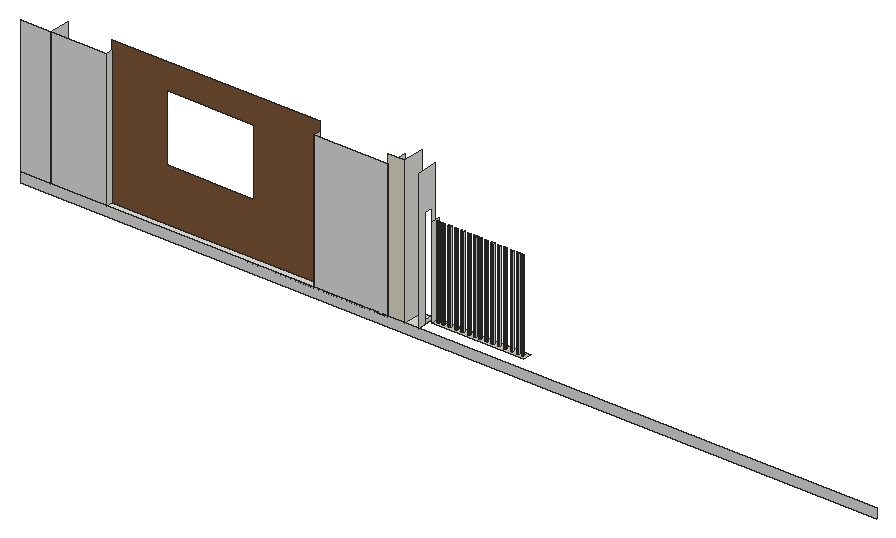
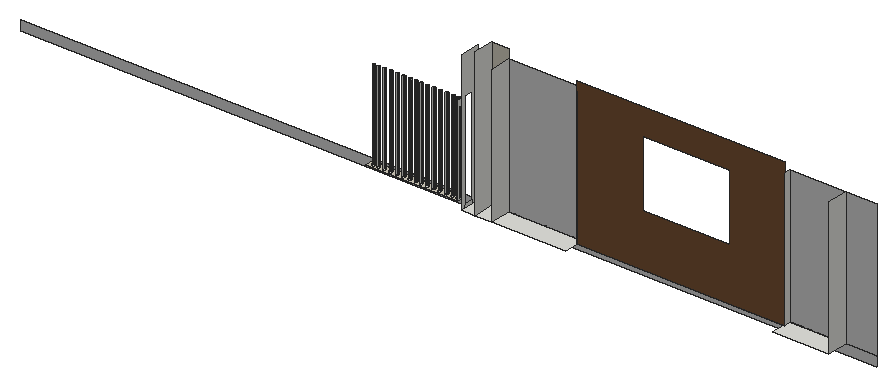
# SketchUp Ruby script. Lengths in inches.
U = 1.inch
M = Sketchup.active_model
def pt(a) = Geom::Point3d.new(a.map { |v| v * U })
def face(e, loops, mat)
  f = e.add_face(loops[0].map { |a| pt(a) })
  loops[1..].each { |l| e.add_face(l.map { |a| pt(a) }).erase! }
  f.material = f.back_material = mat if mat
  f
end
# faces: each face lists its corners as indices into pts; further lists are holes
def faces(e, pts, list, mat = nil) = list.each { |f| face(e, (f[0].is_a?(Array) ? f : [f]).map { |l| l.map { |i| pts[i] } }, mat) }
# xy, xz, yz: faces in a plane at the given z, y or x. An outline is a flat list of corners, or four numbers for a rectangle; further outlines are holes
def ring(l) = l.size == 4 ? [[l[0], l[1]], [l[2], l[1]], [l[2], l[3]], [l[0], l[3]]] : l.each_slice(2).to_a
def flat(e, list, mat, &to3) = list.each { |f| face(e, (f[0].is_a?(Array) ? f : [f]).map { |l| ring(l).map { |u, v| to3.(u, v) } }, mat) }
def xy(e, z, list, mat = nil) = flat(e, list, mat) { |x, y| [x, y, z] }
def xz(e, y, list, mat = nil) = flat(e, list, mat) { |x, z| [x, y, z] }
def yz(e, x, list, mat = nil) = flat(e, list, mat) { |y, z| [x, y, z] }
def lines(e, pts, list) = list.each { |a, b| e.add_line(pt(pts[a]), pt(pts[b])) }
# prism: a flat outline (further loops are holes) pulled along v
def prism(e, loops, v, mat = nil)
  f = face(e, loops, mat); d = Geom::Vector3d.new(v.map { |x| x * U })
  f.pushpull(f.normal.samedirection?(d) ? d.length : -d.length)
end
def box(e, o, s, mat = nil) = prism(e, [[o, [o[0] + s[0], o[1], o[2]], [o[0] + s[0], o[1] + s[1], o[2]], [o[0], o[1] + s[1], o[2]]]], [0, 0, s[2]], mat)
def at(x, y, z, deg = 0) = Geom::Transformation.translation(pt([x, y, z])) * Geom::Transformation.rotation(ORIGIN, Z_AXIS, deg.degrees)
def axes(o, x, y, z) = Geom::Transformation.new([*x, 0, *y, 0, *z, 0, *pt(o).to_a, 1])
def part(name) = M.definitions.add(name)
# library, detail: a bought-in or finely detailed component or shape, given as its bounding box
def library(name, o, s) = part(name).tap { |d| box(d.entities, o, s) }
def detail(e, o, s) = box(e.add_group.entities, o, s)
def put(e, d, t, mat = nil) = e.add_instance(d, t).tap { |i| i.material = mat if mat }
def group(e, t, mat = nil) = e.add_group.tap { |g| g.transformation = t; g.material = mat if mat }.entities
root = M.entities
M.materials.add("[Cladding Siding White]").color = [207, 207, 207]
M.materials.add("[Formica Graystone]").color = [209, 204, 189]
M.materials.add("[Sandstone]").color = [118, 81, 52]
xy(root,9,[[28.1,1.67,80.35,21.38],[80.35,1.67,273.1875,8.25],[273.1875,1.67,342.51,21.38],[342.51,1.67,357.9375,21.38],[357.9375,1.67,370.65,21.38]])
xy(root,12.5,[[380.14,12.51,379.82,12.55,379.52,12.67,379.26,12.875,379.06,13.13,378.94,13.43,378.89,13.76,378.94,14.08,379.06,14.38,379.26,14.64,379.52,14.84,379.82,14.96,380.14,15.01,380.47,14.96,380.77,14.84,381.03,14.64,381.23,14.38,381.35,14.08,381.39,13.76,381.35,13.43,381.23,13.13,381.03,12.875,380.77,12.67,380.47,12.55],[384.7,12.51,384.38,12.55,384.08,12.67,383.82,12.875,383.62,13.13,383.49,13.43,383.45,13.76,383.49,14.08,383.62,14.38,383.82,14.64,384.08,14.84,384.38,14.96,384.7,15.01,385.03,14.96,385.33,14.84,385.59,14.64,385.78,14.38,385.91,14.08,385.95,13.76,385.91,13.43,385.78,13.13,385.59,12.875,385.33,12.67,385.03,12.55],[390.45,12.51,390.13,12.55,389.83,12.67,389.57,12.875,389.37,13.13,389.24,13.43,389.2,13.76,389.24,14.08,389.37,14.38,389.57,14.64,389.83,14.84,390.13,14.96,390.45,15.01,390.78,14.96,391.08,14.84,391.34,14.64,391.53,14.38,391.66,14.08,391.7,13.76,391.66,13.43,391.53,13.13,391.34,12.875,391.08,12.67,390.78,12.55],[396.95,12.51,396.63,12.55,396.33,12.67,396.07,12.875,395.87,13.13,395.74,13.43,395.7,13.76,395.74,14.08,395.87,14.38,396.07,14.64,396.33,14.84,396.63,14.96,396.95,15.01,397.28,14.96,397.58,14.84,397.84,14.64,398.03,14.38,398.16,14.08,398.2,13.76,398.16,13.43,398.03,13.13,397.84,12.875,397.58,12.67,397.28,12.55],[402.58,12.51,402.25,12.55,401.95,12.67,401.69,12.875,401.49,13.13,401.37,13.43,401.33,13.76,401.37,14.08,401.49,14.38,401.69,14.64,401.95,14.84,402.25,14.96,402.58,15.01,402.9,14.96,403.2,14.84,403.46,14.64,403.66,14.38,403.78,14.08,403.83,13.76,403.78,13.43,403.66,13.13,403.46,12.875,403.2,12.67,402.9,12.55],
  [408.45,12.51,408.13,12.55,407.83,12.67,407.57,12.875,407.37,13.13,407.24,13.43,407.2,13.76,407.24,14.08,407.37,14.38,407.57,14.64,407.83,14.84,408.13,14.96,408.45,15.01,408.78,14.96,409.08,14.84,409.34,14.64,409.53,14.38,409.66,14.08,409.7,13.76,409.66,13.43,409.53,13.13,409.34,12.875,409.08,12.67,408.78,12.55],[414.01,12.51,413.69,12.55,413.39,12.67,413.13,12.875,412.93,13.13,412.81,13.43,412.76,13.76,412.81,14.08,412.93,14.38,413.13,14.64,413.39,14.84,413.69,14.96,414.01,15.01,414.34,14.96,414.64,14.84,414.9,14.64,415.1,14.38,415.22,14.08,415.26,13.76,415.22,13.43,415.1,13.13,414.9,12.875,414.64,12.67,414.34,12.55],[418.89,12.51,418.57,12.55,418.26,12.67,418.01,12.875,417.81,13.13,417.68,13.43,417.64,13.76,417.68,14.08,417.81,14.38,418.01,14.64,418.26,14.84,418.57,14.96,418.89,15.01,419.21,14.96,419.51,14.84,419.77,14.64,419.97,14.38,420.1,14.08,420.14,13.76,420.1,13.43,419.97,13.13,419.77,12.875,419.51,12.67,419.21,12.55],[424.64,12.51,424.32,12.55,424.01,12.67,423.76,12.875,423.56,13.13,423.43,13.43,423.39,13.76,423.43,14.08,423.56,14.38,423.76,14.64,424.01,14.84,424.32,14.96,424.64,15.01,424.96,14.96,425.26,14.84,425.52,14.64,425.72,14.38,425.85,14.08,425.89,13.76,425.85,13.43,425.72,13.13,425.52,12.875,425.26,12.67,424.96,12.55],[430.51,12.51,430.19,12.55,429.89,12.67,429.63,12.875,429.43,13.13,429.31,13.43,429.26,13.76,429.31,14.08,429.43,14.38,429.63,14.64,429.89,14.84,430.19,14.96,430.51,15.01,430.84,14.96,431.14,14.84,431.4,14.64,431.6,14.38,431.72,14.08,431.76,13.76,431.72,13.43,431.6,13.13,431.4,12.875,431.14,12.67,430.84,12.55],
  [436.2,12.51,435.88,12.55,435.58,12.67,435.32,12.875,435.12,13.13,434.99,13.43,434.95,13.76,434.99,14.08,435.12,14.38,435.32,14.64,435.58,14.84,435.88,14.96,436.2,15.01,436.53,14.96,436.83,14.84,437.09,14.64,437.28,14.38,437.41,14.08,437.45,13.76,437.41,13.43,437.28,13.13,437.09,12.875,436.83,12.67,436.53,12.55],[442.45,12.51,442.13,12.55,441.83,12.67,441.57,12.875,441.37,13.13,441.24,13.43,441.2,13.76,441.24,14.08,441.37,14.38,441.57,14.64,441.83,14.84,442.13,14.96,442.45,15.01,442.78,14.96,443.08,14.84,443.34,14.64,443.53,14.38,443.66,14.08,443.7,13.76,443.66,13.43,443.53,13.13,443.34,12.875,443.08,12.67,442.78,12.55],[448.45,12.51,448.13,12.55,447.83,12.67,447.57,12.875,447.37,13.13,447.24,13.43,447.2,13.76,447.24,14.08,447.37,14.38,447.57,14.64,447.83,14.84,448.13,14.96,448.45,15.01,448.78,14.96,449.08,14.84,449.34,14.64,449.53,14.38,449.66,14.08,449.7,13.76,449.66,13.43,449.53,13.13,449.34,12.875,449.08,12.67,448.78,12.55],[453.95,12.51,453.63,12.55,453.33,12.67,453.07,12.875,452.87,13.13,452.74,13.43,452.7,13.76,452.74,14.08,452.87,14.38,453.07,14.64,453.33,14.84,453.63,14.96,453.95,15.01,454.28,14.96,454.58,14.84,454.84,14.64,455.03,14.38,455.16,14.08,455.2,13.76,455.16,13.43,455.03,13.13,454.84,12.875,454.58,12.67,454.28,12.55],[458.64,12.51,458.32,12.55,458.01,12.67,457.76,12.875,457.56,13.13,457.43,13.43,457.39,13.76,457.43,14.08,457.56,14.38,457.76,14.64,458.01,14.84,458.32,14.96,458.64,15.01,458.96,14.96,459.26,14.84,459.52,14.64,459.72,14.38,459.85,14.08,459.89,13.76,459.85,13.43,459.72,13.13,459.52,12.875,459.26,12.67,458.96,12.55]])
xy(root,12.5,[[[377.34,9.54,462.5,17.41],[380.14,12.51,379.82,12.55,379.52,12.67,379.26,12.875,379.06,13.13,378.94,13.43,378.89,13.76,378.94,14.08,379.06,14.38,379.26,14.64,379.52,14.84,379.82,14.96,380.14,15.01,380.47,14.96,380.77,14.84,381.03,14.64,381.23,14.38,381.35,14.08,381.39,13.76,381.35,13.43,381.23,13.13,381.03,12.875,380.77,12.67,380.47,12.55],[458.64,12.51,458.32,12.55,458.01,12.67,457.76,12.875,457.56,13.13,457.43,13.43,457.39,13.76,457.43,14.08,457.56,14.38,457.76,14.64,458.01,14.84,458.32,14.96,458.64,15.01,458.96,14.96,459.26,14.84,459.52,14.64,459.72,14.38,459.85,14.08,459.89,13.76,459.85,13.43,459.72,13.13,459.52,12.875,459.26,12.67,458.96,12.55],[384.7,12.51,384.38,12.55,384.08,12.67,383.82,12.875,383.62,13.13,383.49,13.43,383.45,13.76,383.49,14.08,383.62,14.38,383.82,14.64,384.08,14.84,384.38,14.96,384.7,15.01,385.03,14.96,385.33,14.84,385.59,14.64,385.78,14.38,385.91,14.08,385.95,13.76,385.91,13.43,385.78,13.13,385.59,12.875,385.33,12.67,385.03,12.55],[453.95,12.51,453.63,12.55,453.33,12.67,453.07,12.875,452.87,13.13,452.74,13.43,452.7,13.76,452.74,14.08,452.87,14.38,453.07,14.64,453.33,14.84,453.63,14.96,453.95,15.01,454.28,14.96,454.58,14.84,454.84,14.64,455.03,14.38,455.16,14.08,455.2,13.76,455.16,13.43,455.03,13.13,454.84,12.875,454.58,12.67,454.28,12.55],[390.45,12.51,390.13,12.55,389.83,12.67,389.57,12.875,389.37,13.13,389.24,13.43,389.2,13.76,389.24,14.08,389.37,14.38,389.57,14.64,389.83,14.84,390.13,14.96,390.45,15.01,390.78,14.96,391.08,14.84,391.34,14.64,391.53,14.38,391.66,14.08,391.7,13.76,391.66,13.43,391.53,13.13,391.34,12.875,391.08,12.67,390.78,12.55],[448.45,12.51,448.13,12.55,447.83,12.67,447.57,12.875,447.37,13.13,447.24,13.43,447.2,13.76,447.24,14.08,447.37,14.38,447.57,14.64,447.83,14.84,448.13,14.96,448.45,15.01,448.78,14.96,449.08,14.84,449.34,14.64,449.53,14.38,449.66,14.08,449.7,13.76,449.66,13.43,449.53,13.13,449.34,12.875,449.08,12.67,448.78,12.55],[396.95,12.51,396.63,12.55,396.33,12.67,396.07,12.875,395.87,13.13,395.74,13.43,395.7,13.76,395.74,14.08,395.87,14.38,396.07,14.64,396.33,14.84,396.63,14.96,396.95,15.01,397.28,14.96,397.58,14.84,397.84,14.64,398.03,14.38,398.16,14.08,398.2,13.76,398.16,13.43,398.03,13.13,397.84,12.875,397.58,12.67,397.28,12.55],[442.45,12.51,442.13,12.55,441.83,12.67,441.57,12.875,441.37,13.13,441.24,13.43,441.2,13.76,441.24,14.08,441.37,14.38,441.57,14.64,441.83,14.84,442.13,14.96,442.45,15.01,442.78,14.96,443.08,14.84,443.34,14.64,443.53,14.38,443.66,14.08,443.7,13.76,443.66,13.43,443.53,13.13,443.34,12.875,443.08,12.67,442.78,12.55],[402.58,12.51,402.25,12.55,401.95,12.67,401.69,12.875,401.49,13.13,401.37,13.43,401.33,13.76,401.37,14.08,401.49,14.38,401.69,14.64,401.95,14.84,402.25,14.96,402.58,15.01,402.9,14.96,403.2,14.84,403.46,14.64,403.66,14.38,403.78,14.08,403.83,13.76,403.78,13.43,403.66,13.13,403.46,12.875,403.2,12.67,402.9,12.55],[436.2,12.51,435.88,12.55,435.58,12.67,435.32,12.875,435.12,13.13,434.99,13.43,434.95,13.76,434.99,14.08,435.12,14.38,435.32,14.64,435.58,14.84,435.88,14.96,436.2,15.01,436.53,14.96,436.83,14.84,437.09,14.64,437.28,14.38,437.41,14.08,437.45,13.76,437.41,13.43,437.28,13.13,437.09,12.875,436.83,12.67,436.53,12.55],[408.45,12.51,408.13,12.55,407.83,12.67,407.57,12.875,407.37,13.13,407.24,13.43,407.2,13.76,407.24,14.08,407.37,14.38,407.57,14.64,407.83,14.84,408.13,14.96,408.45,15.01,408.78,14.96,409.08,14.84,409.34,14.64,409.53,14.38,409.66,14.08,409.7,13.76,409.66,13.43,409.53,13.13,409.34,12.875,409.08,12.67,408.78,12.55],[430.51,12.51,430.19,12.55,429.89,12.67,429.63,12.875,429.43,13.13,429.31,13.43,429.26,13.76,429.31,14.08,429.43,14.38,429.63,14.64,429.89,14.84,430.19,14.96,430.51,15.01,430.84,14.96,431.14,14.84,431.4,14.64,431.6,14.38,431.72,14.08,431.76,13.76,431.72,13.43,431.6,13.13,431.4,12.875,431.14,12.67,430.84,12.55],[414.01,12.51,413.69,12.55,413.39,12.67,413.13,12.875,412.93,13.13,412.81,13.43,412.76,13.76,412.81,14.08,412.93,14.38,413.13,14.64,413.39,14.84,413.69,14.96,414.01,15.01,414.34,14.96,414.64,14.84,414.9,14.64,415.1,14.38,415.22,14.08,415.26,13.76,415.22,13.43,415.1,13.13,414.9,12.875,414.64,12.67,414.34,12.55],[418.89,12.51,418.57,12.55,418.26,12.67,418.01,12.875,417.81,13.13,417.68,13.43,417.64,13.76,417.68,14.08,417.81,14.38,418.01,14.64,418.26,14.84,418.57,14.96,418.89,15.01,419.21,14.96,419.51,14.84,419.77,14.64,419.97,14.38,420.1,14.08,420.14,13.76,420.1,13.43,419.97,13.13,419.77,12.875,419.51,12.67,419.21,12.55],[424.64,12.51,424.32,12.55,424.01,12.67,423.76,12.875,423.56,13.13,423.43,13.43,423.39,13.76,423.43,14.08,423.56,14.38,423.76,14.64,424.01,14.84,424.32,14.96,424.64,15.01,424.96,14.96,425.26,14.84,425.52,14.64,425.72,14.38,425.85,14.08,425.89,13.76,425.85,13.43,425.72,13.13,425.52,12.875,425.26,12.67,424.96,12.55]]],"[Formica Graystone]")
xz(root,1.67,[[0,0,797.12,9],[0,9,28.1,136.125],[28.1,9,80.35,136.125],[273.1875,9,342.51,136.125]],"[Cladding Siding White]")
xz(root,1.67,[[342.51,9,357.9375,145.125]],"[Formica Graystone]")
xz(root,8.25,[[[80.35,9,273.1875,145.125],[130.9,58.17,212.59,120.61]]],"[Sandstone]")
yz(root,28.1,[[1.67,9,21.38,136.125]])
yz(root,80.35,[[1.67,9,8.25,136.125]])
yz(root,273.1875,[[1.67,9,8.25,136.125]])
yz(root,342.51,[[1.67,9,21.38,136.125]])
yz(root,357.9375,[[1.67,9,21.38,145.125]])
yz(root,370.65,[[1.67,9,9.54,9,9.54,102.25,17.41,102.25,17.41,9,21.38,9,21.38,138.11,1.67,138.11],[9.54,9,17.41,12.5]])
yz(root,377.34,[[9.54,12.5,17.41,96.37]])
p = [[379.52,12.67,12.5],[379.82,12.55,12.5],[379.82,12.55,96.37],[379.52,12.67,96.37],[380.14,12.51,12.5],[380.14,12.51,96.37],
  [380.47,12.55,12.5],[380.47,12.55,96.37],[380.77,12.67,12.5],[380.77,12.67,96.37],[384.08,12.67,12.5],[384.38,12.55,12.5],
  [384.38,12.55,96.37],[384.08,12.67,96.37],[384.7,12.51,12.5],[384.7,12.51,96.37],[385.03,12.55,12.5],[385.03,12.55,96.37],
  [385.33,12.67,12.5],[385.33,12.67,96.37],[389.83,12.67,12.5],[390.13,12.55,12.5],[390.13,12.55,96.37],[389.83,12.67,96.37],
  [390.45,12.51,12.5],[390.45,12.51,96.37],[390.78,12.55,12.5],[390.78,12.55,96.37],[391.08,12.67,12.5],[391.08,12.67,96.37],
  [396.33,12.67,12.5],[396.63,12.55,12.5],[396.63,12.55,96.37],[396.33,12.67,96.37],[396.95,12.51,12.5],[396.95,12.51,96.37],
  [397.28,12.55,12.5],[397.28,12.55,96.37],[397.58,12.67,12.5],[397.58,12.67,96.37],[401.95,12.67,12.5],[402.25,12.55,12.5],
  [402.25,12.55,96.37],[401.95,12.67,96.37],[402.58,12.51,12.5],[402.58,12.51,96.37],[402.9,12.55,12.5],[402.9,12.55,96.37],
  [403.2,12.67,12.5],[403.2,12.67,96.37],[407.83,12.67,12.5],[408.13,12.55,12.5],[408.13,12.55,96.37],[407.83,12.67,96.37],
  [408.45,12.51,12.5],[408.45,12.51,96.37],[408.78,12.55,12.5],[408.78,12.55,96.37],[409.08,12.67,12.5],[409.08,12.67,96.37],
  [413.39,12.67,12.5],[413.69,12.55,12.5],[413.69,12.55,96.37],[413.39,12.67,96.37],[414.01,12.51,12.5],[414.01,12.51,96.37],
  [414.34,12.55,12.5],[414.34,12.55,96.37],[414.64,12.67,12.5],[414.64,12.67,96.37],[418.26,12.67,12.5],[418.57,12.55,12.5],
  [418.57,12.55,96.37],[418.26,12.67,96.37],[418.89,12.51,12.5],[418.89,12.51,96.37],[419.21,12.55,12.5],[419.21,12.55,96.37],
  [419.51,12.67,12.5],[419.51,12.67,96.37],[424.01,12.67,12.5],[424.32,12.55,12.5],[424.32,12.55,96.37],[424.01,12.67,96.37],
  [424.64,12.51,12.5],[424.64,12.51,96.37],[424.96,12.55,12.5],[424.96,12.55,96.37],[425.26,12.67,12.5],[425.26,12.67,96.37],
  [429.89,12.67,12.5],[430.19,12.55,12.5],[430.19,12.55,96.37],[429.89,12.67,96.37],[430.51,12.51,12.5],[430.51,12.51,96.37],
  [430.84,12.55,12.5],[430.84,12.55,96.37],[431.14,12.67,12.5],[431.14,12.67,96.37],[435.58,12.67,12.5],[435.88,12.55,12.5],
  [435.88,12.55,96.37],[435.58,12.67,96.37],[436.2,12.51,12.5],[436.2,12.51,96.37],[436.53,12.55,12.5],[436.53,12.55,96.37],
  [436.83,12.67,12.5],[436.83,12.67,96.37],[441.83,12.67,12.5],[442.13,12.55,12.5],[442.13,12.55,96.37],[441.83,12.67,96.37],
  [442.45,12.51,12.5],[442.45,12.51,96.37],[442.78,12.55,12.5],[442.78,12.55,96.37],[443.08,12.67,12.5],[443.08,12.67,96.37],
  [447.83,12.67,12.5],[448.13,12.55,12.5],[448.13,12.55,96.37],[447.83,12.67,96.37],[448.45,12.51,12.5],[448.45,12.51,96.37],
  [448.78,12.55,12.5],[448.78,12.55,96.37],[449.08,12.67,12.5],[449.08,12.67,96.37],[453.33,12.67,12.5],[453.63,12.55,12.5],
  [453.63,12.55,96.37],[453.33,12.67,96.37],[453.95,12.51,12.5],[453.95,12.51,96.37],[454.28,12.55,12.5],[454.28,12.55,96.37],
  [454.58,12.67,12.5],[454.58,12.67,96.37],[458.01,12.67,12.5],[458.32,12.55,12.5],[458.32,12.55,96.37],[458.01,12.67,96.37],
  [458.64,12.51,12.5],[458.64,12.51,96.37],[458.96,12.55,12.5],[458.96,12.55,96.37],[459.26,12.67,12.5],[459.26,12.67,96.37],
  [379.26,12.875,12.5],[379.26,12.875,96.37],[381.03,12.875,12.5],[381.03,12.875,96.37],[383.82,12.875,12.5],[383.82,12.875,96.37],
  [385.59,12.875,12.5],[385.59,12.875,96.37],[389.57,12.875,12.5],[389.57,12.875,96.37],[391.34,12.875,12.5],[391.34,12.875,96.37],
  [396.07,12.875,12.5],[396.07,12.875,96.37],[397.84,12.875,12.5],[397.84,12.875,96.37],[401.69,12.875,12.5],[401.69,12.875,96.37],
  [403.46,12.875,12.5],[403.46,12.875,96.37],[407.57,12.875,12.5],[407.57,12.875,96.37],[409.34,12.875,12.5],[409.34,12.875,96.37],
  [413.13,12.875,12.5],[413.13,12.875,96.37],[414.9,12.875,12.5],[414.9,12.875,96.37],[418.01,12.875,12.5],[418.01,12.875,96.37],
  [419.77,12.875,12.5],[419.77,12.875,96.37],[423.76,12.875,12.5],[423.76,12.875,96.37],[425.52,12.875,12.5],[425.52,12.875,96.37],
  [429.63,12.875,12.5],[429.63,12.875,96.37],[431.4,12.875,12.5],[431.4,12.875,96.37],[435.32,12.875,12.5],[435.32,12.875,96.37],
  [437.09,12.875,12.5],[437.09,12.875,96.37],[441.57,12.875,12.5],[441.57,12.875,96.37],[443.34,12.875,12.5],[443.34,12.875,96.37],
  [447.57,12.875,12.5],[447.57,12.875,96.37],[449.34,12.875,12.5],[449.34,12.875,96.37],[453.07,12.875,12.5],[453.07,12.875,96.37],
  [454.84,12.875,12.5],[454.84,12.875,96.37],[457.76,12.875,12.5],[457.76,12.875,96.37],[459.52,12.875,12.5],[459.52,12.875,96.37],
  [379.06,13.13,12.5],[379.06,13.13,96.37],[381.23,13.13,12.5],[381.23,13.13,96.37],[383.62,13.13,12.5],[383.62,13.13,96.37],
  [385.78,13.13,12.5],[385.78,13.13,96.37],[389.37,13.13,12.5],[389.37,13.13,96.37],[391.53,13.13,12.5],[391.53,13.13,96.37],
  [395.87,13.13,12.5],[395.87,13.13,96.37],[398.03,13.13,12.5],[398.03,13.13,96.37],[401.49,13.13,12.5],[401.49,13.13,96.37],
  [403.66,13.13,12.5],[403.66,13.13,96.37],[407.37,13.13,12.5],[407.37,13.13,96.37],[409.53,13.13,12.5],[409.53,13.13,96.37],
  [412.93,13.13,12.5],[412.93,13.13,96.37],[415.1,13.13,12.5],[415.1,13.13,96.37],[417.81,13.13,12.5],[417.81,13.13,96.37],
  [419.97,13.13,12.5],[419.97,13.13,96.37],[423.56,13.13,12.5],[423.56,13.13,96.37],[425.72,13.13,12.5],[425.72,13.13,96.37],
  [429.43,13.13,12.5],[429.43,13.13,96.37],[431.6,13.13,12.5],[431.6,13.13,96.37],[435.12,13.13,12.5],[435.12,13.13,96.37],
  [437.28,13.13,12.5],[437.28,13.13,96.37],[441.37,13.13,12.5],[441.37,13.13,96.37],[443.53,13.13,12.5],[443.53,13.13,96.37],
  [447.37,13.13,12.5],[447.37,13.13,96.37],[449.53,13.13,12.5],[449.53,13.13,96.37],[452.87,13.13,12.5],[452.87,13.13,96.37],
  [455.03,13.13,12.5],[455.03,13.13,96.37],[457.56,13.13,12.5],[457.56,13.13,96.37],[459.72,13.13,12.5],[459.72,13.13,96.37],
  [378.94,13.43,12.5],[378.94,13.43,96.37],[381.35,13.43,12.5],[381.35,13.43,96.37],[383.49,13.43,12.5],[383.49,13.43,96.37],
  [385.91,13.43,12.5],[385.91,13.43,96.37],[389.24,13.43,12.5],[389.24,13.43,96.37],[391.66,13.43,12.5],[391.66,13.43,96.37],
  [395.74,13.43,12.5],[395.74,13.43,96.37],[398.16,13.43,12.5],[398.16,13.43,96.37],[401.37,13.43,12.5],[401.37,13.43,96.37],
  [403.78,13.43,12.5],[403.78,13.43,96.37],[407.24,13.43,12.5],[407.24,13.43,96.37],[409.66,13.43,12.5],[409.66,13.43,96.37],
  [412.81,13.43,12.5],[412.81,13.43,96.37],[415.22,13.43,12.5],[415.22,13.43,96.37],[417.68,13.43,12.5],[417.68,13.43,96.37],
  [420.1,13.43,12.5],[420.1,13.43,96.37],[423.43,13.43,12.5],[423.43,13.43,96.37],[425.85,13.43,12.5],[425.85,13.43,96.37],
  [429.31,13.43,12.5],[429.31,13.43,96.37],[431.72,13.43,12.5],[431.72,13.43,96.37],[434.99,13.43,12.5],[434.99,13.43,96.37],
  [437.41,13.43,12.5],[437.41,13.43,96.37],[441.24,13.43,12.5],[441.24,13.43,96.37],[443.66,13.43,12.5],[443.66,13.43,96.37],
  [447.24,13.43,12.5],[447.24,13.43,96.37],[449.66,13.43,12.5],[449.66,13.43,96.37],[452.74,13.43,12.5],[452.74,13.43,96.37],
  [455.16,13.43,12.5],[455.16,13.43,96.37],[457.43,13.43,12.5],[457.43,13.43,96.37],[459.85,13.43,12.5],[459.85,13.43,96.37],
  [378.89,13.76,12.5],[378.89,13.76,96.37],[381.39,13.76,12.5],[381.39,13.76,96.37],[383.45,13.76,12.5],[383.45,13.76,96.37],
  [385.95,13.76,12.5],[385.95,13.76,96.37],[389.2,13.76,12.5],[389.2,13.76,96.37],[391.7,13.76,12.5],[391.7,13.76,96.37],
  [395.7,13.76,12.5],[395.7,13.76,96.37],[398.2,13.76,12.5],[398.2,13.76,96.37],[401.33,13.76,12.5],[401.33,13.76,96.37],
  [403.83,13.76,12.5],[403.83,13.76,96.37],[407.2,13.76,12.5],[407.2,13.76,96.37],[409.7,13.76,12.5],[409.7,13.76,96.37],
  [412.76,13.76,12.5],[412.76,13.76,96.37],[415.26,13.76,12.5],[415.26,13.76,96.37],[417.64,13.76,12.5],[417.64,13.76,96.37],
  [420.14,13.76,12.5],[420.14,13.76,96.37],[423.39,13.76,12.5],[423.39,13.76,96.37],[425.89,13.76,12.5],[425.89,13.76,96.37],
  [429.26,13.76,12.5],[429.26,13.76,96.37],[431.76,13.76,12.5],[431.76,13.76,96.37],[434.95,13.76,12.5],[434.95,13.76,96.37],
  [437.45,13.76,12.5],[437.45,13.76,96.37],[441.2,13.76,12.5],[441.2,13.76,96.37],[443.7,13.76,12.5],[443.7,13.76,96.37],
  [447.2,13.76,12.5],[447.2,13.76,96.37],[449.7,13.76,12.5],[449.7,13.76,96.37],[452.7,13.76,12.5],[452.7,13.76,96.37],
  [455.2,13.76,12.5],[455.2,13.76,96.37],[457.39,13.76,12.5],[457.39,13.76,96.37],[378.94,14.08,12.5],[378.94,14.08,96.37]]
faces(root,p,[[0,1,2,3],[1,4,5,2],[4,6,7,5],[6,8,9,7],[10,11,12,13],[11,14,15,12],[14,16,17,15],[16,18,19,17],
  [20,21,22,23],[21,24,25,22],[24,26,27,25],[26,28,29,27],[30,31,32,33],[31,34,35,32],[34,36,37,35],[36,38,39,37],
  [40,41,42,43],[41,44,45,42],[44,46,47,45],[46,48,49,47],[50,51,52,53],[51,54,55,52],[54,56,57,55],[56,58,59,57],
  [60,61,62,63],[61,64,65,62],[64,66,67,65],[66,68,69,67],[70,71,72,73],[71,74,75,72],[74,76,77,75],[76,78,79,77],
  [80,81,82,83],[81,84,85,82],[84,86,87,85],[86,88,89,87],[90,91,92,93],[91,94,95,92],[94,96,97,95],[96,98,99,97],
  [100,101,102,103],[101,104,105,102],[104,106,107,105],[106,108,109,107],[110,111,112,113],[111,114,115,112],[114,116,117,115],[116,118,119,117],
  [120,121,122,123],[121,124,125,122],[124,126,127,125],[126,128,129,127],[130,131,132,133],[131,134,135,132],[134,136,137,135],[136,138,139,137],
  [140,141,142,143],[141,144,145,142],[144,146,147,145],[146,148,149,147],[150,0,3,151],[8,152,153,9],[154,10,13,155],[18,156,157,19],
  [158,20,23,159],[28,160,161,29],[162,30,33,163],[38,164,165,39],[166,40,43,167],[48,168,169,49],[170,50,53,171],[58,172,173,59],
  [174,60,63,175],[68,176,177,69],[178,70,73,179],[78,180,181,79],[182,80,83,183],[88,184,185,89],[186,90,93,187],[98,188,189,99],
  [190,100,103,191],[108,192,193,109],[194,110,113,195],[118,196,197,119],[198,120,123,199],[128,200,201,129],[202,130,133,203],[138,204,205,139],
  [206,140,143,207],[148,208,209,149],[210,150,151,211],[152,212,213,153],[214,154,155,215],[156,216,217,157],[218,158,159,219],[160,220,221,161],
  [222,162,163,223],[164,224,225,165],[226,166,167,227],[168,228,229,169],[230,170,171,231],[172,232,233,173],[234,174,175,235],[176,236,237,177],
  [238,178,179,239],[180,240,241,181],[242,182,183,243],[184,244,245,185],[246,186,187,247],[188,248,249,189],[250,190,191,251],[192,252,253,193],
  [254,194,195,255],[196,256,257,197],[258,198,199,259],[200,260,261,201],[262,202,203,263],[204,264,265,205],[266,206,207,267],[208,268,269,209],
  [270,210,211,271],[212,272,273,213],[274,214,215,275],[216,276,277,217],[278,218,219,279],[220,280,281,221],[282,222,223,283],[224,284,285,225],
  [286,226,227,287],[228,288,289,229],[290,230,231,291],[232,292,293,233],[294,234,235,295],[236,296,297,237],[298,238,239,299],[240,300,301,241],
  [302,242,243,303],[244,304,305,245],[306,246,247,307],[248,308,309,249],[310,250,251,311],[252,312,313,253],[314,254,255,315],[256,316,317,257],
  [318,258,259,319],[260,320,321,261],[322,262,263,323],[264,324,325,265],[326,266,267,327],[268,328,329,269],[330,270,271,331],[272,332,333,273],
  [334,274,275,335],[276,336,337,277],[338,278,279,339],[280,340,341,281],[342,282,283,343],[284,344,345,285],[346,286,287,347],[288,348,349,289],
  [350,290,291,351],[292,352,353,293],[354,294,295,355],[296,356,357,297],[358,298,299,359],[300,360,361,301],[362,302,303,363],[304,364,365,305],
  [366,306,307,367],[308,368,369,309],[370,310,311,371],[312,372,373,313],[374,314,315,375],[316,376,377,317],[378,318,319,379],[320,380,381,321],
  [382,322,323,383],[324,384,385,325],[386,326,327,387],[388,330,331,389]])
